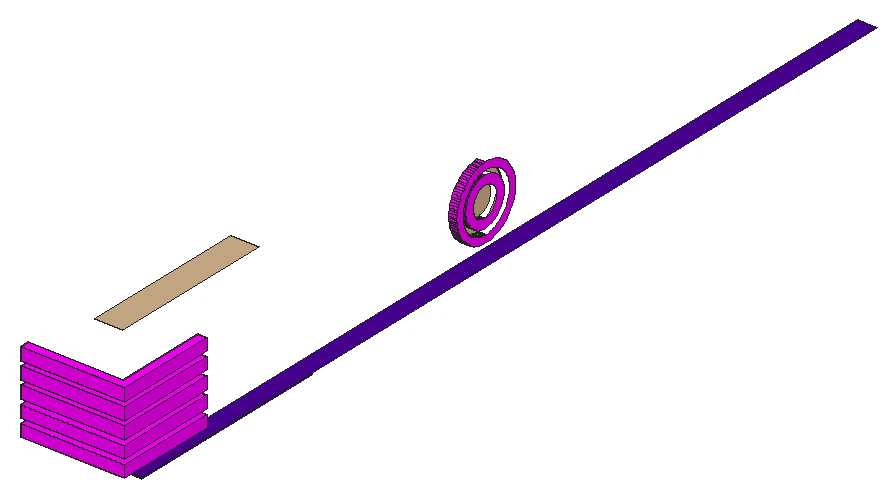
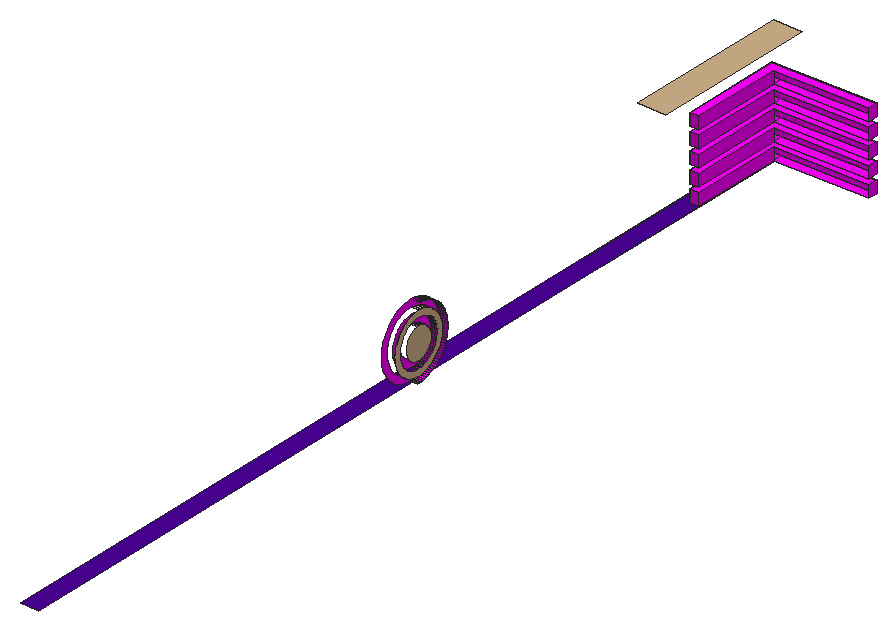
# SketchUp Ruby script. Lengths in inches.
U = 1.inch
M = Sketchup.active_model
def pt(a) = Geom::Point3d.new(a.map { |v| v * U })
def face(e, loops, mat)
  f = e.add_face(loops[0].map { |a| pt(a) })
  loops[1..].each { |l| e.add_face(l.map { |a| pt(a) }).erase! }
  f.material = f.back_material = mat if mat
  f
end
# faces: each face lists its corners as indices into pts; further lists are holes
def faces(e, pts, list, mat = nil) = list.each { |f| face(e, (f[0].is_a?(Array) ? f : [f]).map { |l| l.map { |i| pts[i] } }, mat) }
# xy, xz, yz: faces in a plane at the given z, y or x. An outline is a flat list of corners, or four numbers for a rectangle; further outlines are holes
def ring(l) = l.size == 4 ? [[l[0], l[1]], [l[2], l[1]], [l[2], l[3]], [l[0], l[3]]] : l.each_slice(2).to_a
def flat(e, list, mat, &to3) = list.each { |f| face(e, (f[0].is_a?(Array) ? f : [f]).map { |l| ring(l).map { |u, v| to3.(u, v) } }, mat) }
def xy(e, z, list, mat = nil) = flat(e, list, mat) { |x, y| [x, y, z] }
def xz(e, y, list, mat = nil) = flat(e, list, mat) { |x, z| [x, y, z] }
def yz(e, x, list, mat = nil) = flat(e, list, mat) { |y, z| [x, y, z] }
def lines(e, pts, list) = list.each { |a, b| e.add_line(pt(pts[a]), pt(pts[b])) }
# prism: a flat outline (further loops are holes) pulled along v
def prism(e, loops, v, mat = nil)
  f = face(e, loops, mat); d = Geom::Vector3d.new(v.map { |x| x * U })
  f.pushpull(f.normal.samedirection?(d) ? d.length : -d.length)
end
def box(e, o, s, mat = nil) = prism(e, [[o, [o[0] + s[0], o[1], o[2]], [o[0] + s[0], o[1] + s[1], o[2]], [o[0], o[1] + s[1], o[2]]]], [0, 0, s[2]], mat)
def at(x, y, z, deg = 0) = Geom::Transformation.translation(pt([x, y, z])) * Geom::Transformation.rotation(ORIGIN, Z_AXIS, deg.degrees)
def axes(o, x, y, z) = Geom::Transformation.new([*x, 0, *y, 0, *z, 0, *pt(o).to_a, 1])
def part(name) = M.definitions.add(name)
# library, detail: a bought-in or finely detailed component or shape, given as its bounding box
def library(name, o, s) = part(name).tap { |d| box(d.entities, o, s) }
def detail(e, o, s) = box(e.add_group.entities, o, s)
def put(e, d, t, mat = nil) = e.add_instance(d, t).tap { |i| i.material = mat if mat }
def group(e, t, mat = nil) = e.add_group.tap { |g| g.transformation = t; g.material = mat if mat }.entities
root = M.entities
M.materials.add("[0035_Tan]").color = [210, 180, 140]
M.materials.add("[0127_Magenta]").color = [255, 0, 255]
M.materials.add("[Color J07]").color = [76, 0, 153]
c1 = part("Component\#9")
xy(c1.entities,-20.29,[[-2,0,0,2.5625]],"[0127_Magenta]")
xy(c1.entities,0,[[0,0,19.8125,2.5625]],"[0127_Magenta]")
xy(c1.entities,2,[[-2,0,19.8125,2.5625]],"[0127_Magenta]")
xz(c1.entities,0,[[-2,-20.29,0,0],[-2,0,19.8125,2]],"[0127_Magenta]")
xz(c1.entities,2.5625,[[-2,-20.29,-2,2,19.8125,2,19.8125,0,0,0,0,-20.29]],"[0127_Magenta]")
yz(c1.entities,-2,[[0,-20.29,2.5625,2]],"[0127_Magenta]")
yz(c1.entities,19.8125,[[0,0,2.5625,2]],"[0127_Magenta]")
xy(root,147,[[444,2,448,47.2]])
xy(root,147.28,[[444,2,448,197.1]],"[Color J07]")
xy(root,147.98,[[442,98.5,443.75,98.98]],"[0127_Magenta]")
xy(root,150.68,[[442,98.59,443.5,98.9]],"[0127_Magenta]")
xy(root,152.45,[[442,98.64,443.5,98.85]],"[0035_Tan]")
xy(root,158.9,[[442,98.65,443.5,98.85]],"[0035_Tan]")
xy(root,160.67,[[442,98.6,443.5,98.91]],"[0127_Magenta]")
xy(root,174,[[438,2,444,38]],"[0035_Tan]")
xz(root,2,[[444,147,448,147.28]],"[Color J07]")
xz(root,91.06,[[442,155.4375,443.75,155.92]],"[0127_Magenta]")
xz(root,92.51,[[442,155.48,443.75,155.875]],"[0035_Tan]")
xz(root,93.75,[[442,155.52,443.5,155.84]],"[0127_Magenta]")
xz(root,95.53,[[442,155.57,443.5,155.78]],"[0035_Tan]")
yz(root,442,[[[98.9375,149.43,99.33,149.46,99.72,149.51,100.1,149.58,100.48,149.68,100.86,149.8,101.22,149.94,101.58,150.11,101.92,150.3,102.25,150.51,102.57,150.74,102.87,150.99,103.16,151.26,103.43,151.54,103.68,151.84,103.91,152.16,104.12,152.49,104.31,152.83,104.47,153.1875,104.62,153.55,104.74,153.93,104.84,154.3,104.91,154.69,104.96,155.08,104.99,155.47,104.99,155.86,104.96,156.25,104.91,156.64,104.84,157.03,104.74,157.41,104.625,157.78,104.48,158.15,104.3125,158.5,104.125,158.84,103.92,159.18,103.69,159.49,103.44,159.79,103.17,160.08,102.88,160.35,102.58,160.6,102.26,160.83,101.93,161.04,101.59,161.23,101.23,161.4,100.87,161.54,100.5,161.66,100.12,161.76,99.73,161.84,99.34,161.89,98.95,161.91,98.56,161.91,98.17,161.89,97.78,161.84,97.39,161.76,97.01,161.67,96.64,161.55,96.28,161.4,95.92,161.24,95.58,161.05,95.25,160.84,94.93,160.61,94.63,160.36,94.34,160.09,94.07,159.8,93.82,159.5,93.59,159.1875,93.38,158.86,93.19,158.51,93.02,158.16,92.88,157.79,92.76,157.42,92.66,157.04,92.59,156.66,92.54,156.27,92.51,155.875,92.51,155.48,92.54,155.09,92.58,154.7,92.66,154.32,92.75,153.9375,92.875,153.57,93.02,153.2,93.1875,152.85,93.375,152.5,93.58,152.17,93.8125,151.85,94.0625,151.55,94.33,151.26,94.62,151,94.92,150.75,95.24,150.51,95.57,150.3,95.91,150.12,96.26,149.95,96.63,149.8,97,149.68,97.38,149.58,97.77,149.51,98.16,149.46,98.55,149.44],[98.55,149.46,98.16,149.49,97.77,149.53,97.39,149.61,97.01,149.71,96.64,149.83,96.27,149.97,95.92,150.14,95.58,150.33,95.25,150.54,94.93,150.77,94.63,151.01,94.35,151.28,94.08,151.57,93.83,151.87,93.61,152.18,93.4,152.51,93.21,152.86,93.04,153.21,92.9,153.57,92.78,153.95,92.68,154.32,92.61,154.71,92.5625,155.09,92.54,155.48,92.54,155.875,92.5625,156.26,92.61,156.65,92.69,157.04,92.78,157.41,92.9,157.78,93.05,158.15,93.21,158.5,93.4,158.84,93.61,159.17,93.84,159.49,94.09,159.79,94.36,160.07,94.64,160.34,94.95,160.59,95.26,160.82,95.59,161.03,95.93,161.21,96.29,161.38,96.65,161.52,97.02,161.64,97.4,161.74,97.78,161.8125,98.17,161.86,98.5625,161.89,98.95,161.89,99.34,161.86,99.73,161.8125,100.11,161.74,100.49,161.64,100.86,161.52,101.22,161.375,101.58,161.21,101.92,161.02,102.25,160.81,102.56,160.58,102.87,160.33,103.15,160.0625,103.42,159.78,103.67,159.48,103.89,159.16,104.1,158.83,104.29,158.49,104.46,158.14,104.6,157.77,104.72,157.4,104.82,157.02,104.89,156.64,104.9375,156.25,104.96,155.86,104.96,155.47,104.9375,155.08,104.89,154.69,104.8125,154.31,104.72,153.93,104.6,153.5625,104.45,153.2,104.28,152.84,104.1,152.5,103.89,152.17,103.66,151.86,103.41,151.56,103.14,151.27,102.86,151.01,102.55,150.76,102.24,150.53,101.91,150.32,101.57,150.13,101.21,149.97,100.85,149.82,100.48,149.7,100.1,149.61,99.72,149.53,99.33,149.48,98.9375,149.46]],[[98.55,149.46,98.9375,149.46,99.33,149.48,99.72,149.53,100.1,149.61,100.48,149.7,100.85,149.82,101.21,149.97,101.57,150.13,101.91,150.32,102.24,150.53,102.55,150.76,102.86,151.01,103.14,151.27,103.41,151.56,103.66,151.86,103.89,152.17,104.1,152.5,104.28,152.84,104.45,153.2,104.6,153.5625,104.72,153.93,104.8125,154.31,104.89,154.69,104.9375,155.08,104.96,155.47,104.96,155.86,104.9375,156.25,104.89,156.64,104.82,157.02,104.72,157.4,104.6,157.77,104.46,158.14,104.29,158.49,104.1,158.83,103.89,159.16,103.67,159.48,103.42,159.78,103.15,160.0625,102.87,160.33,102.56,160.58,102.25,160.81,101.92,161.02,101.58,161.21,101.22,161.375,100.86,161.52,100.49,161.64,100.11,161.74,99.73,161.8125,99.34,161.86,98.95,161.89,98.5625,161.89,98.17,161.86,97.78,161.8125,97.4,161.74,97.02,161.64,96.65,161.52,96.29,161.38,95.93,161.21,95.59,161.03,95.26,160.82,94.95,160.59,94.64,160.34,94.36,160.07,94.09,159.79,93.84,159.49,93.61,159.17,93.4,158.84,93.21,158.5,93.05,158.15,92.9,157.78,92.78,157.41,92.69,157.04,92.61,156.65,92.5625,156.26,92.54,155.875,92.54,155.48,92.5625,155.09,92.61,154.71,92.68,154.32,92.78,153.95,92.9,153.57,93.04,153.21,93.21,152.86,93.4,152.51,93.61,152.18,93.83,151.87,94.08,151.57,94.35,151.28,94.63,151.01,94.93,150.77,95.25,150.54,95.58,150.33,95.92,150.14,96.27,149.97,96.64,149.83,97.01,149.71,97.39,149.61,97.77,149.53,98.16,149.49],[98.59,150.68,98.27,150.7,97.96,150.74,97.65,150.79,97.35,150.87,97.05,150.97,96.76,151.09,96.47,151.22,96.2,151.37,95.93,151.54,95.68,151.73,95.4375,151.93,95.21,152.14,95,152.37,94.8,152.61,94.61,152.87,94.44,153.13,94.29,153.41,94.16,153.69,94.04,153.98,93.95,154.28,93.87,154.59,93.81,154.9,93.77,155.21,93.75,155.52,93.75,155.84,93.77,156.15,93.8125,156.46,93.87,156.77,93.95,157.07,94.05,157.37,94.16,157.66,94.3,157.95,94.45,158.22,94.62,158.49,94.8,158.74,95,158.98,95.22,159.21,95.45,159.43,95.6875,159.625,95.94,159.8125,96.21,159.98,96.48,160.13,96.77,160.26,97.0625,160.38,97.36,160.48,97.66,160.55,97.97,160.61,98.28,160.65,98.6,160.67,98.91,160.67,99.23,160.65,99.54,160.61,99.85,160.55,100.15,160.47,100.45,160.375,100.74,160.26,101.02,160.125,101.3,159.97,101.5625,159.81,101.82,159.62,102.06,159.42,102.29,159.2,102.5,158.98,102.7,158.73,102.89,158.48,103.06,158.21,103.21,157.9375,103.34,157.65,103.46,157.36,103.55,157.0625,103.63,156.76,103.6875,156.45,103.73,156.14,103.75,155.82,103.75,155.51,103.73,155.2,103.6875,154.89,103.63,154.58,103.55,154.27,103.45,153.97,103.34,153.68,103.2,153.4,103.05,153.12,102.88,152.86,102.7,152.6,102.5,152.36,102.28,152.13,102.05,151.92,101.81,151.72,101.56,151.53,101.29,151.37,101.01,151.22,100.73,151.08,100.4375,150.97,100.14,150.87,99.84,150.79,99.53,150.73,99.21,150.69,98.9,150.68]],[98.64,152.45,98.85,152.45,99.05,152.46,99.45,152.52,99.65,152.57,100.03,152.71,100.21,152.8,100.39,152.9,100.56,153,100.72,153.12,100.88,153.25,101.03,153.39,101.17,153.54,101.3,153.69,101.52,154.03,101.62,154.21,101.71,154.39,101.85,154.77,101.9,154.97,101.93,155.16,101.96,155.37,101.97,155.57,101.97,155.77,101.96,155.97,101.94,156.17,101.9,156.37,101.85,156.57,101.71,156.95,101.625,157.13,101.53,157.3125,101.42,157.48,101.3,157.65,101.17,157.8,101.03,157.95,100.88,158.09,100.73,158.22,100.57,158.34,100.39,158.45,100.22,158.54,100.03,158.63,99.85,158.71,99.65,158.77,99.46,158.82,99.26,158.86,99.06,158.88,98.85,158.9,98.65,158.9,98.25,158.86,98.05,158.82,97.85,158.77,97.66,158.71,97.47,158.63,97.29,158.55,97.11,158.45,96.94,158.34,96.78,158.22,96.62,158.09,96.47,157.96,96.33,157.81,96.2,157.65,96.08,157.49,95.98,157.32,95.88,157.14,95.79,156.96,95.65,156.58,95.6,156.38,95.54,155.98,95.53,155.78,95.53,155.57,95.54,155.37,95.5625,155.17,95.6,154.97,95.65,154.78,95.71,154.58,95.79,154.4,95.875,154.21,95.97,154.03,96.08,153.86,96.2,153.7,96.33,153.54,96.47,153.39,96.61,153.26,96.77,153.125,96.93,153.01,97.11,152.9,97.28,152.8,97.47,152.71,97.65,152.64,97.85,152.58,98.04,152.53,98.24,152.49,98.44,152.46]],"[0035_Tan]")
yz(root,443.5,[[[98.59,150.68,98.9,150.68,99.21,150.69,99.53,150.73,99.84,150.79,100.14,150.87,100.4375,150.97,100.73,151.08,101.01,151.22,101.29,151.37,101.56,151.53,101.81,151.72,102.05,151.92,102.28,152.13,102.5,152.36,102.7,152.6,102.88,152.86,103.05,153.12,103.2,153.4,103.34,153.68,103.45,153.97,103.55,154.27,103.63,154.58,103.6875,154.89,103.73,155.2,103.75,155.51,103.75,155.82,103.73,156.14,103.6875,156.45,103.63,156.76,103.55,157.0625,103.46,157.36,103.34,157.65,103.21,157.9375,103.06,158.21,102.89,158.48,102.7,158.73,102.5,158.98,102.29,159.2,102.06,159.42,101.82,159.62,101.5625,159.81,101.3,159.97,101.02,160.125,100.74,160.26,100.45,160.375,100.15,160.47,99.85,160.55,99.54,160.61,99.23,160.65,98.91,160.67,98.6,160.67,98.28,160.65,97.97,160.61,97.66,160.55,97.36,160.48,97.0625,160.38,96.77,160.26,96.48,160.13,96.21,159.98,95.94,159.8125,95.6875,159.625,95.45,159.43,95.22,159.21,95,158.98,94.8,158.74,94.62,158.49,94.45,158.22,94.3,157.95,94.16,157.66,94.05,157.37,93.95,157.07,93.87,156.77,93.8125,156.46,93.77,156.15,93.75,155.84,93.75,155.52,93.77,155.21,93.81,154.9,93.87,154.59,93.95,154.28,94.04,153.98,94.16,153.69,94.29,153.41,94.44,153.13,94.61,152.87,94.8,152.61,95,152.37,95.21,152.14,95.4375,151.93,95.68,151.73,95.93,151.54,96.2,151.37,96.47,151.22,96.76,151.09,97.05,150.97,97.35,150.87,97.65,150.79,97.96,150.74,98.27,150.7],[98.64,152.45,98.44,152.46,98.24,152.49,98.04,152.53,97.85,152.58,97.65,152.64,97.47,152.71,97.28,152.8,97.11,152.9,96.93,153.01,96.77,153.125,96.61,153.26,96.47,153.39,96.33,153.54,96.2,153.7,96.08,153.86,95.97,154.03,95.875,154.21,95.79,154.4,95.71,154.58,95.65,154.78,95.6,154.97,95.5625,155.17,95.54,155.37,95.53,155.57,95.53,155.78,95.54,155.98,95.6,156.38,95.65,156.58,95.79,156.96,95.88,157.14,95.98,157.32,96.08,157.49,96.2,157.65,96.33,157.81,96.47,157.96,96.62,158.09,96.78,158.22,96.94,158.34,97.11,158.45,97.29,158.55,97.47,158.63,97.66,158.71,97.85,158.77,98.05,158.82,98.25,158.86,98.65,158.9,98.85,158.9,99.06,158.88,99.26,158.86,99.46,158.82,99.65,158.77,99.85,158.71,100.03,158.63,100.22,158.54,100.39,158.45,100.57,158.34,100.73,158.22,100.88,158.09,101.03,157.95,101.17,157.8,101.3,157.65,101.42,157.48,101.53,157.3125,101.625,157.13,101.71,156.95,101.85,156.57,101.9,156.37,101.94,156.17,101.96,155.97,101.97,155.77,101.97,155.57,101.96,155.37,101.93,155.16,101.9,154.97,101.85,154.77,101.71,154.39,101.62,154.21,101.52,154.03,101.3,153.69,101.17,153.54,101.03,153.39,100.88,153.25,100.72,153.12,100.56,153,100.39,152.9,100.21,152.8,100.03,152.71,99.65,152.57,99.45,152.52,99.05,152.46,98.85,152.45]]],"[0127_Magenta]")
yz(root,443.75,[[[98.5,147.98,98.98,147.98,99.47,148.01,99.95,148.07,100.42,148.16,100.89,148.28,101.35,148.43,101.8,148.61,102.24,148.8125,102.66,149.04,103.07,149.3,103.46,149.59,103.83,149.89,104.1875,150.22,104.52,150.58,104.83,150.95,105.11,151.34,105.37,151.75,105.6,152.17,105.81,152.61,105.99,153.06,106.14,153.52,106.26,153.99,106.35,154.46,106.41,154.94,106.44,155.42,106.44,155.91,106.41,156.39,106.35,156.87,106.26,157.34,106.14,157.8125,105.99,158.27,105.82,158.72,105.61,159.16,105.38,159.58,105.12,159.99,104.84,160.38,104.53,160.76,104.2,161.11,103.85,161.44,103.47,161.75,103.08,162.03,102.67,162.29,102.25,162.53,101.8125,162.73,101.36,162.91,100.9,163.0625,100.4375,163.18,99.96,163.27,99.48,163.33,99,163.37,98.52,163.37,98.03,163.34,97.55,163.28,97.08,163.1875,96.61,163.07,96.15,162.92,95.7,162.74,95.26,162.53,94.84,162.3,94.43,162.04,94.04,161.76,93.67,161.45,93.3125,161.12,92.98,160.77,92.67,160.4,92.39,160.01,92.13,159.6,91.9,159.17,91.69,158.74,91.51,158.29,91.36,157.83,91.24,157.36,91.15,156.88,91.09,156.41,91.06,155.92,91.06,155.4375,91.09,154.96,91.15,154.48,91.24,154,91.36,153.53,91.51,153.07,91.68,152.625,91.89,152.1875,92.12,151.76,92.38,151.35,92.66,150.96,92.97,150.59,93.3,150.24,93.65,149.91,94.03,149.6,94.42,149.3125,94.82,149.05,95.25,148.82,95.69,148.61,96.13,148.43,96.59,148.28,97.0625,148.16,97.54,148.07,98.02,148.01],[98.9375,149.43,98.55,149.44,98.16,149.46,97.77,149.51,97.38,149.58,97,149.68,96.63,149.8,96.26,149.95,95.91,150.12,95.57,150.3,95.24,150.51,94.92,150.75,94.62,151,94.33,151.26,94.0625,151.55,93.8125,151.85,93.58,152.17,93.375,152.5,93.1875,152.85,93.02,153.2,92.875,153.57,92.75,153.9375,92.66,154.32,92.58,154.7,92.54,155.09,92.51,155.48,92.51,155.875,92.54,156.27,92.59,156.66,92.66,157.04,92.76,157.42,92.88,157.79,93.02,158.16,93.19,158.51,93.38,158.86,93.59,159.1875,93.82,159.5,94.07,159.8,94.34,160.09,94.63,160.36,94.93,160.61,95.25,160.84,95.58,161.05,95.92,161.24,96.28,161.4,96.64,161.55,97.01,161.67,97.39,161.76,97.78,161.84,98.17,161.89,98.56,161.91,98.95,161.91,99.34,161.89,99.73,161.84,100.12,161.76,100.5,161.66,100.87,161.54,101.23,161.4,101.59,161.23,101.93,161.04,102.26,160.83,102.58,160.6,102.88,160.35,103.17,160.08,103.44,159.79,103.69,159.49,103.92,159.18,104.125,158.84,104.3125,158.5,104.48,158.15,104.625,157.78,104.74,157.41,104.84,157.03,104.91,156.64,104.96,156.25,104.99,155.86,104.99,155.47,104.96,155.08,104.91,154.69,104.84,154.3,104.74,153.93,104.62,153.55,104.47,153.1875,104.31,152.83,104.12,152.49,103.91,152.16,103.68,151.84,103.43,151.54,103.16,151.26,102.87,150.99,102.57,150.74,102.25,150.51,101.92,150.3,101.58,150.11,101.22,149.94,100.86,149.8,100.48,149.68,100.1,149.58,99.72,149.51,99.33,149.46]]],"[0127_Magenta]")
yz(root,448,[[2,147,47.2,147.28]],"[Color J07]")
p = [[442,97.54,148.07],[442,98.02,148.01],[443.75,98.02,148.01],[443.75,97.54,148.07],[442,98.5,147.98],[443.75,98.5,147.98],
  [442,97.0625,148.16],[443.75,97.0625,148.16],[442,96.59,148.28],[443.75,96.59,148.28],[442,96.13,148.43],[443.75,96.13,148.43],
  [442,95.69,148.61],[443.75,95.69,148.61],[442,95.25,148.82],[443.75,95.25,148.82],[442,94.82,149.05],[443.75,94.82,149.05],
  [442,94.42,149.3125],[443.75,94.42,149.3125],[442,94.03,149.6],[443.75,94.03,149.6],[442,98.55,149.44],[442,98.16,149.46],
  [443.75,98.16,149.46],[443.75,98.55,149.44],[442,98.9375,149.43],[443.75,98.9375,149.43],[442,97.77,149.51],[442,97.38,149.58],
  [443.75,97.38,149.58],[443.75,97.77,149.51],[442,93.65,149.91],[443.75,93.65,149.91],[442,97,149.68],[443.75,97,149.68],
  [442,96.63,149.8],[443.75,96.63,149.8],[442,96.26,149.95],[443.75,96.26,149.95],[442,93.3,150.24],[443.75,93.3,150.24],
  [442,95.91,150.12],[443.75,95.91,150.12],[442,95.57,150.3],[443.75,95.57,150.3],[442,92.97,150.59],[443.75,92.97,150.59],
  [442,95.24,150.51],[443.75,95.24,150.51],[442,94.92,150.75],[443.75,94.92,150.75],[442,92.66,150.96],[443.75,92.66,150.96],
  [442,94.62,151],[443.75,94.62,151],[442,97.65,150.79],[442,97.96,150.74],[443.5,97.96,150.74],[443.5,97.65,150.79],
  [442,98.27,150.7],[443.5,98.27,150.7],[442,98.59,150.68],[443.5,98.59,150.68],[442,97.35,150.87],[443.5,97.35,150.87],
  [442,97.05,150.97],[443.5,97.05,150.97],[442,92.38,151.35],[443.75,92.38,151.35],[442,94.33,151.26],[443.75,94.33,151.26],
  [442,96.76,151.09],[443.5,96.76,151.09],[442,96.47,151.22],[443.5,96.47,151.22],[442,96.2,151.37],[443.5,96.2,151.37],
  [442,94.0625,151.55],[443.75,94.0625,151.55],[442,92.12,151.76],[443.75,92.12,151.76],[442,95.93,151.54],[443.5,95.93,151.54],
  [442,95.68,151.73],[443.5,95.68,151.73],[442,93.8125,151.85],[443.75,93.8125,151.85],[442,95.4375,151.93],[443.5,95.4375,151.93],
  [442,91.89,152.1875],[443.75,91.89,152.1875],[442,93.58,152.17],[443.75,93.58,152.17],[442,95.21,152.14],[443.5,95.21,152.14],
  [442,95,152.37],[443.5,95,152.37],[442,91.68,152.625],[443.75,91.68,152.625],[442,93.375,152.5],[443.75,93.375,152.5],
  [442,94.8,152.61],[443.5,94.8,152.61],[442,98.64,152.45],[442,98.44,152.46],[443.5,98.44,152.46],[443.5,98.64,152.45],
  [442,93.1875,152.85],[443.75,93.1875,152.85],[442,98.04,152.53],[442,97.85,152.58],[443.5,97.85,152.58],[443.5,98.04,152.53],
  [442,98.24,152.49],[443.5,98.24,152.49],[442,91.51,153.07],[443.75,91.51,153.07],[442,94.61,152.87],[443.5,94.61,152.87],
  [442,97.65,152.64],[442,97.47,152.71],[443.5,97.47,152.71],[443.5,97.65,152.64],[442,97.28,152.8],[443.5,97.28,152.8],
  [442,93.02,153.2],[443.75,93.02,153.2],[442,97.11,152.9],[443.5,97.11,152.9],[442,94.44,153.13],[443.5,94.44,153.13],
  [442,96.93,153.01],[443.5,96.93,153.01],[442,96.77,153.125],[443.5,96.77,153.125],[442,91.36,153.53],[443.75,91.36,153.53],
  [442,94.29,153.41],[443.5,94.29,153.41],[442,96.61,153.26],[443.5,96.61,153.26],[442,92.875,153.57],[443.75,92.875,153.57],
  [442,96.47,153.39],[443.5,96.47,153.39],[442,94.16,153.69],[443.5,94.16,153.69],[442,96.33,153.54],[443.5,96.33,153.54],
  [442,91.24,154],[443.75,91.24,154],[442,96.2,153.7],[443.5,96.2,153.7],[442,92.75,153.9375],[443.75,92.75,153.9375],
  [442,94.04,153.98],[443.5,94.04,153.98],[442,96.08,153.86],[443.5,96.08,153.86],[442,92.66,154.32],[443.75,92.66,154.32],
  [442,95.97,154.03],[443.5,95.97,154.03],[442,91.15,154.48],[443.75,91.15,154.48],[442,93.95,154.28],[443.5,93.95,154.28],
  [442,95.875,154.21],[443.5,95.875,154.21],[442,95.79,154.4],[443.5,95.79,154.4],[442,92.58,154.7],[443.75,92.58,154.7],
  [442,93.87,154.59],[443.5,93.87,154.59],[442,95.71,154.58],[443.5,95.71,154.58],[442,91.09,154.96],[443.75,91.09,154.96],
  [442,93.81,154.9],[443.5,93.81,154.9],[442,95.65,154.78],[443.5,95.65,154.78],[442,92.54,155.09],[443.75,92.54,155.09],
  [442,95.6,154.97],[443.5,95.6,154.97],[442,93.77,155.21],[443.5,93.77,155.21],[442,91.06,155.4375],[443.75,91.06,155.4375],
  [442,95.5625,155.17],[443.5,95.5625,155.17],[442,92.51,155.48],[443.75,92.51,155.48],[442,93.75,155.52],[443.5,93.75,155.52],
  [442,95.54,155.37],[443.5,95.54,155.37],[442,95.53,155.57],[443.5,95.53,155.57],[442,93.77,156.15],[442,93.75,155.84],
  [443.5,93.75,155.84],[443.5,93.77,156.15],[442,95.53,155.78],[442,95.54,155.98],[443.5,95.54,155.98],[443.5,95.53,155.78],
  [442,91.09,156.41],[442,91.06,155.92],[443.75,91.06,155.92],[443.75,91.09,156.41],[442,92.51,155.875],[442,92.54,156.27],
  [443.75,92.54,156.27],[443.75,92.51,155.875],[442,95.57,156.18],[443.5,95.57,156.18],[442,93.8125,156.46],[443.5,93.8125,156.46],
  [442,95.6,156.38],[443.5,95.6,156.38],[442,92.59,156.66],[443.75,92.59,156.66],[442,91.15,156.88],[443.75,91.15,156.88],
  [442,95.65,156.58],[443.5,95.65,156.58],[442,93.87,156.77],[443.5,93.87,156.77],[442,95.72,156.77],[443.5,95.72,156.77],
  [442,92.66,157.04],[443.75,92.66,157.04],[442,93.95,157.07],[443.5,93.95,157.07],[442,95.79,156.96],[443.5,95.79,156.96],
  [442,91.24,157.36],[443.75,91.24,157.36],[442,92.76,157.42],[443.75,92.76,157.42],[442,95.88,157.14],[443.5,95.88,157.14],
  [442,94.05,157.37],[443.5,94.05,157.37],[442,95.98,157.32],[443.5,95.98,157.32],[442,96.08,157.49],[443.5,96.08,157.49],
  [442,91.36,157.83],[443.75,91.36,157.83],[442,92.88,157.79],[443.75,92.88,157.79],[442,94.16,157.66],[443.5,94.16,157.66],
  [442,96.2,157.65],[443.5,96.2,157.65],[442,94.3,157.95],[443.5,94.3,157.95],[442,96.33,157.81],[443.5,96.33,157.81],
  [442,91.51,158.29],[443.75,91.51,158.29],[442,93.02,158.16],[443.75,93.02,158.16],[442,96.47,157.96],[443.5,96.47,157.96],
  [442,94.45,158.22],[443.5,94.45,158.22],[442,96.62,158.09],[443.5,96.62,158.09],[442,96.78,158.22],[443.5,96.78,158.22],
  [442,93.19,158.51],[443.75,93.19,158.51],[442,94.62,158.49],[443.5,94.62,158.49],[442,96.94,158.34],[443.5,96.94,158.34],
  [442,91.69,158.74],[443.75,91.69,158.74],[442,97.11,158.45],[443.5,97.11,158.45],[442,93.38,158.86],[443.75,93.38,158.86],
  [442,94.8,158.74],[443.5,94.8,158.74],[442,97.29,158.55],[443.5,97.29,158.55],[442,97.47,158.63],[443.5,97.47,158.63],
  [442,97.66,158.71],[443.5,97.66,158.71],[442,91.9,159.17],[443.75,91.9,159.17],[442,95,158.98],[443.5,95,158.98],
  [442,97.85,158.77],[443.5,97.85,158.77],[442,98.05,158.82],[443.5,98.05,158.82],[442,98.25,158.86],[443.5,98.25,158.86],
  [442,93.59,159.1875],[443.75,93.59,159.1875],[442,98.45,158.88],[443.5,98.45,158.88],[442,98.65,158.9],[443.5,98.65,158.9],
  [442,95.22,159.21],[443.5,95.22,159.21],[442,92.13,159.6],[443.75,92.13,159.6],[442,93.82,159.5],[443.75,93.82,159.5],
  [442,95.45,159.43],[443.5,95.45,159.43],[442,95.6875,159.625],[443.5,95.6875,159.625],[442,94.07,159.8],[443.75,94.07,159.8],
  [442,92.39,160.01],[443.75,92.39,160.01],[442,95.94,159.8125],[443.5,95.94,159.8125],[442,94.34,160.09],[443.75,94.34,160.09],
  [442,96.21,159.98],[443.5,96.21,159.98],[442,92.67,160.4],[443.75,92.67,160.4],[442,96.48,160.13],[443.5,96.48,160.13],
  [442,94.63,160.36],[443.75,94.63,160.36],[442,96.77,160.26],[443.5,96.77,160.26],[442,97.0625,160.38],[443.5,97.0625,160.38],
  [442,92.98,160.77],[443.75,92.98,160.77],[442,94.93,160.61],[443.75,94.93,160.61],[442,97.36,160.48],[443.5,97.36,160.48],
  [442,97.66,160.55],[443.5,97.66,160.55],[442,95.25,160.84],[443.75,95.25,160.84],[442,97.97,160.61],[443.5,97.97,160.61],
  [442,98.28,160.65],[443.5,98.28,160.65],[442,98.6,160.67],[443.5,98.6,160.67],[442,93.3125,161.12],[443.75,93.3125,161.12],
  [442,95.58,161.05],[443.75,95.58,161.05],[442,95.92,161.24],[443.75,95.92,161.24],[442,93.67,161.45],[443.75,93.67,161.45],
  [442,96.28,161.4],[443.75,96.28,161.4],[442,96.64,161.55],[443.75,96.64,161.55],[442,94.04,161.76],[443.75,94.04,161.76],
  [442,97.01,161.67],[443.75,97.01,161.67],[442,97.39,161.76],[443.75,97.39,161.76],[442,94.43,162.04],[443.75,94.43,162.04],
  [442,97.78,161.84],[443.75,97.78,161.84],[442,98.17,161.89],[443.75,98.17,161.89],[442,98.56,161.91],[443.75,98.56,161.91],
  [442,94.84,162.3],[443.75,94.84,162.3],[442,95.26,162.53],[443.75,95.26,162.53],[442,95.7,162.74],[443.75,95.7,162.74],
  [442,96.15,162.92],[443.75,96.15,162.92],[442,96.61,163.07],[443.75,96.61,163.07],[442,97.08,163.1875],[443.75,97.08,163.1875],
  [442,97.55,163.28],[443.75,97.55,163.28],[442,98.03,163.34],[443.75,98.03,163.34],[442,98.52,163.37],[443.75,98.52,163.37]]
faces(root,p,[[0,1,2,3],[1,4,5,2],[6,0,3,7],[8,6,7,9],[10,8,9,11],[12,10,11,13],[14,12,13,15],[16,14,15,17],
  [18,16,17,19],[20,18,19,21],[32,20,21,33],[40,32,33,41],[46,40,41,47],[52,46,47,53],[56,57,58,59],[57,60,61,58],
  [60,62,63,61],[64,56,59,65],[66,64,65,67],[68,52,53,69],[72,66,67,73],[74,72,73,75],[76,74,75,77],[80,68,69,81],
  [82,76,77,83],[84,82,83,85],[88,84,85,89],[90,80,81,91],[94,88,89,95],[96,94,95,97],[98,90,91,99],[102,96,97,103],
  [116,98,99,117],[118,102,103,119],[130,118,119,131],[136,116,117,137],[138,130,131,139],[146,138,139,147],[150,136,137,151],[156,146,147,157],
  [164,150,151,165],[166,156,157,167],[174,166,167,175],[178,164,165,179],[180,174,175,181],[188,180,181,189],[190,178,179,191],[196,188,189,197],
  [202,203,204,205],[210,211,212,213],[220,202,205,221],[226,210,213,227],[230,220,221,231],[236,230,231,237],[240,226,227,241],[246,236,237,247],
  [252,240,241,253],[256,246,247,257],[260,256,257,261],[264,252,253,265],[270,260,261,271],[278,270,271,279],[282,264,265,283],[288,278,279,289],
  [296,282,283,297],[298,288,289,299],[312,298,299,313],[314,296,297,315],[318,312,313,319],[320,318,319,321],[324,314,315,325],[326,320,321,327],
  [330,326,327,331],[332,324,325,333],[334,330,331,335],[338,334,335,339],[340,338,339,341],[342,332,333,343],[346,340,341,347],[348,346,347,349],
  [352,348,349,353],[354,352,353,355],[356,354,355,357],[358,342,343,359],[364,358,359,365],[370,364,365,371],[376,370,371,377],[384,376,377,385],
  [386,384,385,387],[388,386,387,389],[390,388,389,391],[392,390,391,393],[394,392,393,395],[396,394,395,397],[398,396,397,399],[400,398,399,401]],"[0127_Magenta]")
faces(root,p,[[22,23,24,25],[26,22,25,27],[28,29,30,31],[23,28,31,24],[29,34,35,30],[34,36,37,35],[36,38,39,37],[38,42,43,39],
  [42,44,45,43],[44,48,49,45],[48,50,51,49],[50,54,55,51],[54,70,71,55],[70,78,79,71],[78,86,87,79],[86,92,93,87],
  [92,100,101,93],[104,105,106,107],[100,108,109,101],[110,111,112,113],[114,110,113,115],[105,114,115,106],[120,121,122,123],[111,120,123,112],
  [121,124,125,122],[108,126,127,109],[124,128,129,125],[128,132,133,129],[132,134,135,133],[134,140,141,135],[126,142,143,127],[140,144,145,141],
  [144,148,149,145],[148,152,153,149],[142,154,155,143],[152,158,159,153],[154,160,161,155],[158,162,163,159],[162,168,169,163],[168,170,171,169],
  [160,172,173,161],[170,176,177,171],[176,182,183,177],[172,184,185,173],[182,186,187,183],[186,192,193,187],[184,194,195,185],[192,198,199,193],
  [198,200,201,199],[206,207,208,209],[214,215,216,217],[207,218,219,208],[218,222,223,219],[215,224,225,216],[222,228,229,223],[228,232,233,229],
  [224,234,235,225],[232,238,239,233],[234,242,243,235],[238,244,245,239],[244,248,249,245],[248,250,251,249],[242,254,255,243],[250,258,259,251],
  [258,262,263,259],[254,266,267,255],[262,268,269,263],[268,272,273,269],[272,274,275,273],[266,276,277,267],[274,280,281,275],[280,284,285,281],
  [276,286,287,277],[284,290,291,285],[290,292,293,291],[292,294,295,293],[294,300,301,295],[300,302,303,301],[302,304,305,303],[286,306,307,287],
  [304,308,309,305],[308,310,311,309],[306,316,317,307],[316,322,323,317],[322,328,329,323],[328,336,337,329],[336,344,345,337],[344,350,351,345],
  [350,360,361,351],[360,362,363,361],[362,366,367,363],[366,368,369,367],[368,372,373,369],[372,374,375,373],[374,378,379,375],[378,380,381,379],
  [380,382,383,381]],"[0035_Tan]")
put(root,c1,axes([444,2,147.28],[0,1,0],[0,0,1],[1,0,0]),"[0127_Magenta]")
put(root,c1,axes([444,2,150.93],[0,1,0],[0,0,1],[1,0,0]),"[0127_Magenta]")
put(root,c1,axes([444,2,154.58],[0,1,0],[0,0,1],[1,0,0]),"[0127_Magenta]")
put(root,c1,axes([444,2,158.23],[0,1,0],[0,0,1],[1,0,0]),"[0127_Magenta]")
put(root,c1,axes([444,2,161.875],[0,1,0],[0,0,1],[1,0,0]),"[0127_Magenta]")
